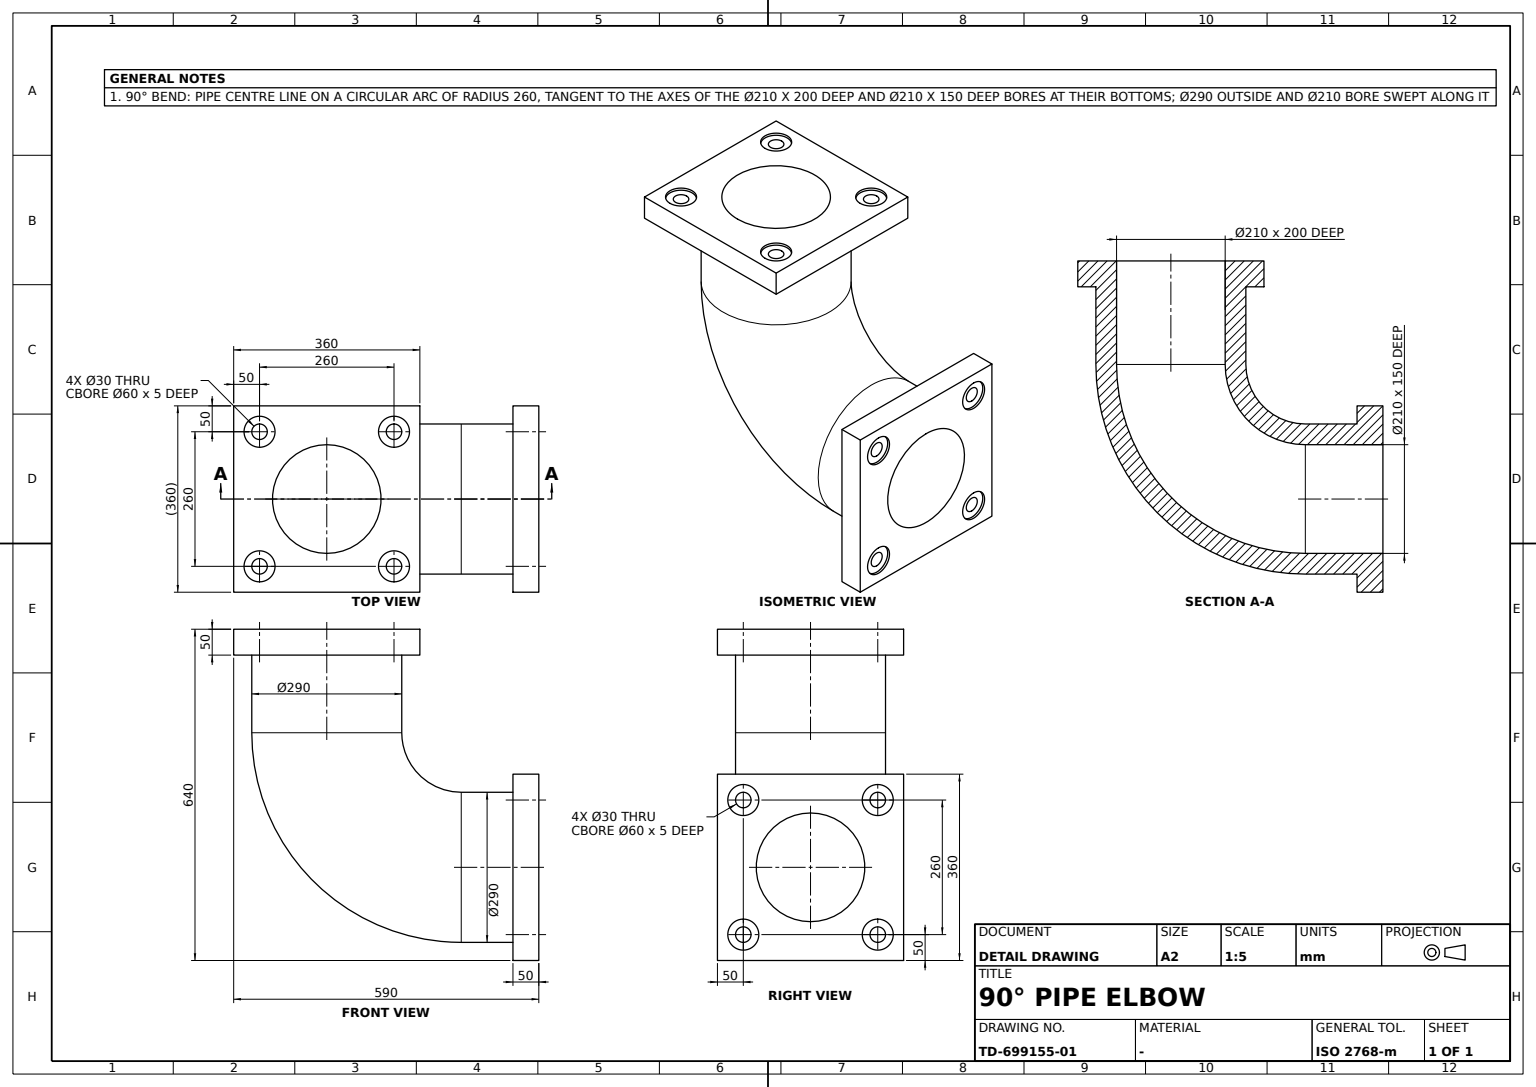
ISO-10303-21;
HEADER;
FILE_DESCRIPTION((''),'2;1');
FILE_NAME('','',(''),(''),'','','');
FILE_SCHEMA(('AUTOMOTIVE_DESIGN'));
ENDSEC;
DATA;
#1=APPLICATION_CONTEXT('');
#2=PRODUCT_CONTEXT('',#1,'mechanical');
#3=PRODUCT('','','',(#2));
#4=PRODUCT_DEFINITION_FORMATION('','',#3);
#5=PRODUCT_DEFINITION_CONTEXT('',#1,'design');
#6=PRODUCT_DEFINITION('','',#4,#5);
#7=PRODUCT_DEFINITION_SHAPE('','',#6);
#8=(LENGTH_UNIT()NAMED_UNIT(*)SI_UNIT(.MILLI.,.METRE.));
#9=(NAMED_UNIT(*)PLANE_ANGLE_UNIT()SI_UNIT($,.RADIAN.));
#10=(NAMED_UNIT(*)SI_UNIT($,.STERADIAN.)SOLID_ANGLE_UNIT());
#11=UNCERTAINTY_MEASURE_WITH_UNIT(LENGTH_MEASURE(0.005),#8,'distance_accuracy_value','');
#12=(GEOMETRIC_REPRESENTATION_CONTEXT(3)GLOBAL_UNCERTAINTY_ASSIGNED_CONTEXT((#11))GLOBAL_UNIT_ASSIGNED_CONTEXT((#8,#9,#10))REPRESENTATION_CONTEXT('',''));
#13=CARTESIAN_POINT('',(160.,-130.,460.));
#14=VERTEX_POINT('',#13);
#15=CARTESIAN_POINT('',(130.,-130.,460.));
#16=DIRECTION('',(0.,0.,1.));
#17=DIRECTION('',(1.,0.,0.));
#18=AXIS2_PLACEMENT_3D('',#15,#16,#17);
#19=CIRCLE('',#18,30.);
#20=EDGE_CURVE('',#14,#14,#19,.T.);
#21=ORIENTED_EDGE('',*,*,#20,.F.);
#22=EDGE_LOOP('',(#21));
#23=FACE_BOUND('',#22,.T.);
#24=CARTESIAN_POINT('',(105.,0.,460.));
#25=VERTEX_POINT('',#24);
#26=CARTESIAN_POINT('',(0.,0.,460.));
#27=AXIS2_PLACEMENT_3D('',#26,#16,#17);
#28=CIRCLE('',#27,105.);
#29=EDGE_CURVE('',#25,#25,#28,.T.);
#30=ORIENTED_EDGE('',*,*,#29,.F.);
#31=EDGE_LOOP('',(#30));
#32=FACE_BOUND('',#31,.T.);
#33=CARTESIAN_POINT('',(160.,130.,460.));
#34=VERTEX_POINT('',#33);
#35=CARTESIAN_POINT('',(130.,130.,460.));
#36=AXIS2_PLACEMENT_3D('',#35,#16,#17);
#37=CIRCLE('',#36,30.);
#38=EDGE_CURVE('',#34,#34,#37,.T.);
#39=ORIENTED_EDGE('',*,*,#38,.F.);
#40=EDGE_LOOP('',(#39));
#41=FACE_BOUND('',#40,.T.);
#42=CARTESIAN_POINT('',(-100.,130.,460.));
#43=VERTEX_POINT('',#42);
#44=CARTESIAN_POINT('',(-130.,130.,460.));
#45=AXIS2_PLACEMENT_3D('',#44,#16,#17);
#46=CIRCLE('',#45,30.);
#47=EDGE_CURVE('',#43,#43,#46,.T.);
#48=ORIENTED_EDGE('',*,*,#47,.F.);
#49=EDGE_LOOP('',(#48));
#50=FACE_BOUND('',#49,.T.);
#51=CARTESIAN_POINT('',(-180.,180.,460.));
#52=VERTEX_POINT('',#51);
#53=CARTESIAN_POINT('',(180.,180.,460.));
#54=VERTEX_POINT('',#53);
#55=CARTESIAN_POINT('',(0.,180.,460.));
#56=VECTOR('',#17,1000.);
#57=LINE('',#55,#56);
#58=EDGE_CURVE('',#52,#54,#57,.T.);
#59=ORIENTED_EDGE('',*,*,#58,.F.);
#60=CARTESIAN_POINT('',(-180.,-180.,460.));
#61=VERTEX_POINT('',#60);
#62=CARTESIAN_POINT('',(-180.,410.,460.));
#63=DIRECTION('',(0.,1.,0.));
#64=VECTOR('',#63,1000.);
#65=LINE('',#62,#64);
#66=EDGE_CURVE('',#61,#52,#65,.T.);
#67=ORIENTED_EDGE('',*,*,#66,.F.);
#68=CARTESIAN_POINT('',(180.,-180.,460.));
#69=VERTEX_POINT('',#68);
#70=CARTESIAN_POINT('',(0.,-180.,460.));
#71=DIRECTION('',(-1.,0.,0.));
#72=VECTOR('',#71,1000.);
#73=LINE('',#70,#72);
#74=EDGE_CURVE('',#69,#61,#73,.T.);
#75=ORIENTED_EDGE('',*,*,#74,.F.);
#76=CARTESIAN_POINT('',(180.,410.,460.));
#77=DIRECTION('',(0.,-1.,0.));
#78=VECTOR('',#77,1000.);
#79=LINE('',#76,#78);
#80=EDGE_CURVE('',#54,#69,#79,.T.);
#81=ORIENTED_EDGE('',*,*,#80,.F.);
#82=EDGE_LOOP('',(#59,#67,#75,#81));
#83=FACE_BOUND('',#82,.T.);
#84=CARTESIAN_POINT('',(-100.,-130.,460.));
#85=VERTEX_POINT('',#84);
#86=CARTESIAN_POINT('',(-130.,-130.,460.));
#87=AXIS2_PLACEMENT_3D('',#86,#16,#17);
#88=CIRCLE('',#87,30.);
#89=EDGE_CURVE('',#85,#85,#88,.T.);
#90=ORIENTED_EDGE('',*,*,#89,.F.);
#91=EDGE_LOOP('',(#90));
#92=FACE_BOUND('',#91,.T.);
#93=PLANE('',#27);
#94=ADVANCED_FACE('',(#23,#32,#41,#50,#83,#92),#93,.T.);
#95=CARTESIAN_POINT('',(-180.,410.,-180.));
#96=VERTEX_POINT('',#95);
#97=CARTESIAN_POINT('',(180.,410.,-180.));
#98=VERTEX_POINT('',#97);
#99=LINE('',#95,#56);
#100=EDGE_CURVE('',#96,#98,#99,.T.);
#101=ORIENTED_EDGE('',*,*,#100,.T.);
#102=CARTESIAN_POINT('',(180.,360.,-180.));
#103=VERTEX_POINT('',#102);
#104=LINE('',#97,#78);
#105=EDGE_CURVE('',#98,#103,#104,.T.);
#106=ORIENTED_EDGE('',*,*,#105,.T.);
#107=CARTESIAN_POINT('',(-180.,360.,-180.));
#108=VERTEX_POINT('',#107);
#109=LINE('',#107,#56);
#110=EDGE_CURVE('',#108,#103,#109,.T.);
#111=ORIENTED_EDGE('',*,*,#110,.F.);
#112=LINE('',#95,#78);
#113=EDGE_CURVE('',#96,#108,#112,.T.);
#114=ORIENTED_EDGE('',*,*,#113,.F.);
#115=EDGE_LOOP('',(#101,#106,#111,#114));
#116=FACE_BOUND('',#115,.T.);
#117=DIRECTION('',(0.,0.,-1.));
#118=AXIS2_PLACEMENT_3D('',#95,#117,#17);
#119=PLANE('',#118);
#120=ADVANCED_FACE('',(#116),#119,.T.);
#121=ORIENTED_EDGE('',*,*,#38,.T.);
#122=EDGE_LOOP('',(#121));
#123=FACE_BOUND('',#122,.T.);
#124=CARTESIAN_POINT('',(100.,130.,455.));
#125=VERTEX_POINT('',#124);
#126=CARTESIAN_POINT('',(130.,130.,455.));
#127=AXIS2_PLACEMENT_3D('',#126,#117,#71);
#128=CIRCLE('',#127,30.);
#129=EDGE_CURVE('',#125,#125,#128,.T.);
#130=ORIENTED_EDGE('',*,*,#129,.T.);
#131=EDGE_LOOP('',(#130));
#132=FACE_BOUND('',#131,.T.);
#133=CARTESIAN_POINT('',(130.,130.,459.9));
#134=AXIS2_PLACEMENT_3D('',#133,#117,#17);
#135=CYLINDRICAL_SURFACE('',#134,30.);
#136=ADVANCED_FACE('',(#123,#132),#135,.F.);
#137=CARTESIAN_POINT('',(115.,130.,410.));
#138=VERTEX_POINT('',#137);
#139=CARTESIAN_POINT('',(130.,130.,410.));
#140=AXIS2_PLACEMENT_3D('',#139,#117,#71);
#141=CIRCLE('',#140,15.);
#142=EDGE_CURVE('',#138,#138,#141,.T.);
#143=ORIENTED_EDGE('',*,*,#142,.T.);
#144=EDGE_LOOP('',(#143));
#145=FACE_BOUND('',#144,.T.);
#146=CARTESIAN_POINT('',(115.,130.,455.));
#147=VERTEX_POINT('',#146);
#148=CIRCLE('',#127,15.);
#149=EDGE_CURVE('',#147,#147,#148,.T.);
#150=ORIENTED_EDGE('',*,*,#149,.F.);
#151=EDGE_LOOP('',(#150));
#152=FACE_BOUND('',#151,.T.);
#153=CYLINDRICAL_SURFACE('',#134,15.);
#154=ADVANCED_FACE('',(#145,#152),#153,.F.);
#155=CARTESIAN_POINT('',(-130.,405.,-160.));
#156=VERTEX_POINT('',#155);
#157=CARTESIAN_POINT('',(-130.,405.,-130.));
#158=AXIS2_PLACEMENT_3D('',#157,#77,#117);
#159=CIRCLE('',#158,30.);
#160=EDGE_CURVE('',#156,#156,#159,.T.);
#161=ORIENTED_EDGE('',*,*,#160,.T.);
#162=EDGE_LOOP('',(#161));
#163=FACE_BOUND('',#162,.T.);
#164=CARTESIAN_POINT('',(-130.,410.,-100.));
#165=VERTEX_POINT('',#164);
#166=CARTESIAN_POINT('',(-130.,410.,-130.));
#167=AXIS2_PLACEMENT_3D('',#166,#63,#16);
#168=CIRCLE('',#167,30.);
#169=EDGE_CURVE('',#165,#165,#168,.T.);
#170=ORIENTED_EDGE('',*,*,#169,.T.);
#171=EDGE_LOOP('',(#170));
#172=FACE_BOUND('',#171,.T.);
#173=CARTESIAN_POINT('',(-130.,409.9,-130.));
#174=AXIS2_PLACEMENT_3D('',#173,#77,#17);
#175=CYLINDRICAL_SURFACE('',#174,30.);
#176=ADVANCED_FACE('',(#163,#172),#175,.F.);
#177=CARTESIAN_POINT('',(180.,410.,180.));
#178=VERTEX_POINT('',#177);
#179=VECTOR('',#16,1000.);
#180=LINE('',#97,#179);
#181=EDGE_CURVE('',#98,#178,#180,.T.);
#182=ORIENTED_EDGE('',*,*,#181,.T.);
#183=CARTESIAN_POINT('',(180.,360.,180.));
#184=VERTEX_POINT('',#183);
#185=LINE('',#177,#78);
#186=EDGE_CURVE('',#178,#184,#185,.T.);
#187=ORIENTED_EDGE('',*,*,#186,.T.);
#188=LINE('',#102,#179);
#189=EDGE_CURVE('',#103,#184,#188,.T.);
#190=ORIENTED_EDGE('',*,*,#189,.F.);
#191=ORIENTED_EDGE('',*,*,#105,.F.);
#192=EDGE_LOOP('',(#182,#187,#190,#191));
#193=FACE_BOUND('',#192,.T.);
#194=AXIS2_PLACEMENT_3D('',#97,#17,#16);
#195=PLANE('',#194);
#196=ADVANCED_FACE('',(#193),#195,.T.);
#197=CARTESIAN_POINT('',(0.,260.,105.));
#198=VERTEX_POINT('',#197);
#199=CARTESIAN_POINT('',(0.,260.,0.));
#200=AXIS2_PLACEMENT_3D('',#199,#63,#16);
#201=CIRCLE('',#200,105.);
#202=EDGE_CURVE('',#198,#198,#201,.T.);
#203=ORIENTED_EDGE('',*,*,#202,.F.);
#204=EDGE_LOOP('',(#203));
#205=FACE_BOUND('',#204,.T.);
#206=CARTESIAN_POINT('',(0.,410.,105.));
#207=VERTEX_POINT('',#206);
#208=CARTESIAN_POINT('',(0.,410.,0.));
#209=AXIS2_PLACEMENT_3D('',#208,#63,#16);
#210=CIRCLE('',#209,105.);
#211=EDGE_CURVE('',#207,#207,#210,.T.);
#212=ORIENTED_EDGE('',*,*,#211,.T.);
#213=EDGE_LOOP('',(#212));
#214=FACE_BOUND('',#213,.T.);
#215=CARTESIAN_POINT('',(0.,335.,0.));
#216=AXIS2_PLACEMENT_3D('',#215,#63,#71);
#217=CYLINDRICAL_SURFACE('',#216,105.);
#218=ADVANCED_FACE('',(#205,#214),#217,.F.);
#219=CARTESIAN_POINT('',(-160.,130.,455.));
#220=VERTEX_POINT('',#219);
#221=CARTESIAN_POINT('',(-130.,130.,455.));
#222=AXIS2_PLACEMENT_3D('',#221,#117,#71);
#223=CIRCLE('',#222,30.);
#224=EDGE_CURVE('',#220,#220,#223,.T.);
#225=ORIENTED_EDGE('',*,*,#224,.F.);
#226=EDGE_LOOP('',(#225));
#227=FACE_BOUND('',#226,.T.);
#228=CARTESIAN_POINT('',(-145.,130.,455.));
#229=VERTEX_POINT('',#228);
#230=CIRCLE('',#222,15.);
#231=EDGE_CURVE('',#229,#229,#230,.T.);
#232=ORIENTED_EDGE('',*,*,#231,.T.);
#233=EDGE_LOOP('',(#232));
#234=FACE_BOUND('',#233,.T.);
#235=CARTESIAN_POINT('',(145.,130.,455.));
#236=AXIS2_PLACEMENT_3D('',#235,#117,#17);
#237=PLANE('',#236);
#238=ADVANCED_FACE('',(#227,#234),#237,.F.);
#239=CARTESIAN_POINT('',(-160.,-130.,455.));
#240=VERTEX_POINT('',#239);
#241=CARTESIAN_POINT('',(-130.,-130.,455.));
#242=AXIS2_PLACEMENT_3D('',#241,#117,#71);
#243=CIRCLE('',#242,30.);
#244=EDGE_CURVE('',#240,#240,#243,.T.);
#245=ORIENTED_EDGE('',*,*,#244,.F.);
#246=EDGE_LOOP('',(#245));
#247=FACE_BOUND('',#246,.T.);
#248=CARTESIAN_POINT('',(-145.,-130.,455.));
#249=VERTEX_POINT('',#248);
#250=CIRCLE('',#242,15.);
#251=EDGE_CURVE('',#249,#249,#250,.T.);
#252=ORIENTED_EDGE('',*,*,#251,.T.);
#253=EDGE_LOOP('',(#252));
#254=FACE_BOUND('',#253,.T.);
#255=ADVANCED_FACE('',(#247,#254),#237,.F.);
#256=CARTESIAN_POINT('',(-180.,180.,410.));
#257=VERTEX_POINT('',#256);
#258=CARTESIAN_POINT('',(-180.,180.,180.));
#259=LINE('',#258,#179);
#260=EDGE_CURVE('',#257,#52,#259,.T.);
#261=ORIENTED_EDGE('',*,*,#260,.F.);
#262=CARTESIAN_POINT('',(-180.,-180.,410.));
#263=VERTEX_POINT('',#262);
#264=CARTESIAN_POINT('',(-180.,0.,410.));
#265=LINE('',#264,#64);
#266=EDGE_CURVE('',#263,#257,#265,.T.);
#267=ORIENTED_EDGE('',*,*,#266,.F.);
#268=LINE('',#262,#179);
#269=EDGE_CURVE('',#263,#61,#268,.T.);
#270=ORIENTED_EDGE('',*,*,#269,.T.);
#271=ORIENTED_EDGE('',*,*,#66,.T.);
#272=EDGE_LOOP('',(#261,#267,#270,#271));
#273=FACE_BOUND('',#272,.T.);
#274=CARTESIAN_POINT('',(-180.,410.,180.));
#275=AXIS2_PLACEMENT_3D('',#274,#71,#117);
#276=PLANE('',#275);
#277=ADVANCED_FACE('',(#273),#276,.T.);
#278=CARTESIAN_POINT('',(0.,260.,145.));
#279=VERTEX_POINT('',#278);
#280=CIRCLE('',#200,145.);
#281=EDGE_CURVE('',#279,#279,#280,.T.);
#282=ORIENTED_EDGE('',*,*,#281,.T.);
#283=EDGE_LOOP('',(#282));
#284=FACE_BOUND('',#283,.T.);
#285=CARTESIAN_POINT('',(0.,360.,145.));
#286=VERTEX_POINT('',#285);
#287=CARTESIAN_POINT('',(0.,360.,0.));
#288=AXIS2_PLACEMENT_3D('',#287,#63,#16);
#289=CIRCLE('',#288,145.);
#290=EDGE_CURVE('',#286,#286,#289,.T.);
#291=ORIENTED_EDGE('',*,*,#290,.F.);
#292=EDGE_LOOP('',(#291));
#293=FACE_BOUND('',#292,.T.);
#294=CYLINDRICAL_SURFACE('',#216,145.);
#295=ADVANCED_FACE('',(#284,#293),#294,.T.);
#296=CARTESIAN_POINT('',(-130.,405.,100.));
#297=VERTEX_POINT('',#296);
#298=CARTESIAN_POINT('',(-130.,405.,130.));
#299=AXIS2_PLACEMENT_3D('',#298,#77,#117);
#300=CIRCLE('',#299,30.);
#301=EDGE_CURVE('',#297,#297,#300,.T.);
#302=ORIENTED_EDGE('',*,*,#301,.T.);
#303=EDGE_LOOP('',(#302));
#304=FACE_BOUND('',#303,.T.);
#305=CARTESIAN_POINT('',(-130.,410.,160.));
#306=VERTEX_POINT('',#305);
#307=CARTESIAN_POINT('',(-130.,410.,130.));
#308=AXIS2_PLACEMENT_3D('',#307,#63,#16);
#309=CIRCLE('',#308,30.);
#310=EDGE_CURVE('',#306,#306,#309,.T.);
#311=ORIENTED_EDGE('',*,*,#310,.T.);
#312=EDGE_LOOP('',(#311));
#313=FACE_BOUND('',#312,.T.);
#314=CARTESIAN_POINT('',(-130.,409.9,130.));
#315=AXIS2_PLACEMENT_3D('',#314,#77,#17);
#316=CYLINDRICAL_SURFACE('',#315,30.);
#317=ADVANCED_FACE('',(#304,#313),#316,.F.);
#318=CARTESIAN_POINT('',(115.,-130.,455.));
#319=VERTEX_POINT('',#318);
#320=CARTESIAN_POINT('',(130.,-130.,455.));
#321=AXIS2_PLACEMENT_3D('',#320,#117,#71);
#322=CIRCLE('',#321,15.);
#323=EDGE_CURVE('',#319,#319,#322,.T.);
#324=ORIENTED_EDGE('',*,*,#323,.F.);
#325=EDGE_LOOP('',(#324));
#326=FACE_BOUND('',#325,.T.);
#327=CARTESIAN_POINT('',(115.,-130.,410.));
#328=VERTEX_POINT('',#327);
#329=CARTESIAN_POINT('',(130.,-130.,410.));
#330=AXIS2_PLACEMENT_3D('',#329,#117,#71);
#331=CIRCLE('',#330,15.);
#332=EDGE_CURVE('',#328,#328,#331,.T.);
#333=ORIENTED_EDGE('',*,*,#332,.T.);
#334=EDGE_LOOP('',(#333));
#335=FACE_BOUND('',#334,.T.);
#336=CARTESIAN_POINT('',(130.,-130.,459.9));
#337=AXIS2_PLACEMENT_3D('',#336,#117,#17);
#338=CYLINDRICAL_SURFACE('',#337,15.);
#339=ADVANCED_FACE('',(#326,#335),#338,.F.);
#340=CARTESIAN_POINT('',(130.,405.,-160.));
#341=VERTEX_POINT('',#340);
#342=CARTESIAN_POINT('',(130.,405.,-130.));
#343=AXIS2_PLACEMENT_3D('',#342,#77,#117);
#344=CIRCLE('',#343,30.);
#345=EDGE_CURVE('',#341,#341,#344,.T.);
#346=ORIENTED_EDGE('',*,*,#345,.T.);
#347=EDGE_LOOP('',(#346));
#348=FACE_BOUND('',#347,.T.);
#349=CARTESIAN_POINT('',(130.,410.,-100.));
#350=VERTEX_POINT('',#349);
#351=CARTESIAN_POINT('',(130.,410.,-130.));
#352=AXIS2_PLACEMENT_3D('',#351,#63,#16);
#353=CIRCLE('',#352,30.);
#354=EDGE_CURVE('',#350,#350,#353,.T.);
#355=ORIENTED_EDGE('',*,*,#354,.T.);
#356=EDGE_LOOP('',(#355));
#357=FACE_BOUND('',#356,.T.);
#358=CARTESIAN_POINT('',(130.,409.9,-130.));
#359=AXIS2_PLACEMENT_3D('',#358,#77,#17);
#360=CYLINDRICAL_SURFACE('',#359,30.);
#361=ADVANCED_FACE('',(#348,#357),#360,.F.);
#362=CARTESIAN_POINT('',(-130.,405.,-145.));
#363=VERTEX_POINT('',#362);
#364=CIRCLE('',#158,15.);
#365=EDGE_CURVE('',#363,#363,#364,.T.);
#366=ORIENTED_EDGE('',*,*,#365,.F.);
#367=EDGE_LOOP('',(#366));
#368=FACE_BOUND('',#367,.T.);
#369=CARTESIAN_POINT('',(-130.,360.,-115.));
#370=VERTEX_POINT('',#369);
#371=CARTESIAN_POINT('',(-130.,360.,-130.));
#372=AXIS2_PLACEMENT_3D('',#371,#63,#16);
#373=CIRCLE('',#372,15.);
#374=EDGE_CURVE('',#370,#370,#373,.T.);
#375=ORIENTED_EDGE('',*,*,#374,.F.);
#376=EDGE_LOOP('',(#375));
#377=FACE_BOUND('',#376,.T.);
#378=CYLINDRICAL_SURFACE('',#174,15.);
#379=ADVANCED_FACE('',(#368,#377),#378,.F.);
#380=ORIENTED_EDGE('',*,*,#323,.T.);
#381=EDGE_LOOP('',(#380));
#382=FACE_BOUND('',#381,.T.);
#383=CARTESIAN_POINT('',(100.,-130.,455.));
#384=VERTEX_POINT('',#383);
#385=CIRCLE('',#321,30.);
#386=EDGE_CURVE('',#384,#384,#385,.T.);
#387=ORIENTED_EDGE('',*,*,#386,.F.);
#388=EDGE_LOOP('',(#387));
#389=FACE_BOUND('',#388,.T.);
#390=ADVANCED_FACE('',(#382,#389),#237,.F.);
#391=CARTESIAN_POINT('',(130.,360.,145.));
#392=VERTEX_POINT('',#391);
#393=CARTESIAN_POINT('',(130.,360.,130.));
#394=AXIS2_PLACEMENT_3D('',#393,#63,#16);
#395=CIRCLE('',#394,15.);
#396=EDGE_CURVE('',#392,#392,#395,.T.);
#397=ORIENTED_EDGE('',*,*,#396,.F.);
#398=EDGE_LOOP('',(#397));
#399=FACE_BOUND('',#398,.T.);
#400=CARTESIAN_POINT('',(130.,405.,115.));
#401=VERTEX_POINT('',#400);
#402=CARTESIAN_POINT('',(130.,405.,130.));
#403=AXIS2_PLACEMENT_3D('',#402,#77,#117);
#404=CIRCLE('',#403,15.);
#405=EDGE_CURVE('',#401,#401,#404,.T.);
#406=ORIENTED_EDGE('',*,*,#405,.F.);
#407=EDGE_LOOP('',(#406));
#408=FACE_BOUND('',#407,.T.);
#409=CARTESIAN_POINT('',(130.,409.9,130.));
#410=AXIS2_PLACEMENT_3D('',#409,#77,#17);
#411=CYLINDRICAL_SURFACE('',#410,15.);
#412=ADVANCED_FACE('',(#399,#408),#411,.F.);
#413=ORIENTED_EDGE('',*,*,#244,.T.);
#414=EDGE_LOOP('',(#413));
#415=FACE_BOUND('',#414,.T.);
#416=ORIENTED_EDGE('',*,*,#89,.T.);
#417=EDGE_LOOP('',(#416));
#418=FACE_BOUND('',#417,.T.);
#419=CARTESIAN_POINT('',(-130.,-130.,459.9));
#420=AXIS2_PLACEMENT_3D('',#419,#117,#17);
#421=CYLINDRICAL_SURFACE('',#420,30.);
#422=ADVANCED_FACE('',(#415,#418),#421,.F.);
#423=ORIENTED_EDGE('',*,*,#224,.T.);
#424=EDGE_LOOP('',(#423));
#425=FACE_BOUND('',#424,.T.);
#426=ORIENTED_EDGE('',*,*,#47,.T.);
#427=EDGE_LOOP('',(#426));
#428=FACE_BOUND('',#427,.T.);
#429=CARTESIAN_POINT('',(-130.,130.,459.9));
#430=AXIS2_PLACEMENT_3D('',#429,#117,#17);
#431=CYLINDRICAL_SURFACE('',#430,30.);
#432=ADVANCED_FACE('',(#425,#428),#431,.F.);
#433=CARTESIAN_POINT('',(-145.,130.,410.));
#434=VERTEX_POINT('',#433);
#435=CARTESIAN_POINT('',(-130.,130.,410.));
#436=AXIS2_PLACEMENT_3D('',#435,#117,#71);
#437=CIRCLE('',#436,15.);
#438=EDGE_CURVE('',#434,#434,#437,.T.);
#439=ORIENTED_EDGE('',*,*,#438,.T.);
#440=EDGE_LOOP('',(#439));
#441=FACE_BOUND('',#440,.T.);
#442=ORIENTED_EDGE('',*,*,#231,.F.);
#443=EDGE_LOOP('',(#442));
#444=FACE_BOUND('',#443,.T.);
#445=CYLINDRICAL_SURFACE('',#430,15.);
#446=ADVANCED_FACE('',(#441,#444),#445,.F.);
#447=CARTESIAN_POINT('',(180.,180.,410.));
#448=VERTEX_POINT('',#447);
#449=CARTESIAN_POINT('',(180.,-180.,410.));
#450=VERTEX_POINT('',#449);
#451=CARTESIAN_POINT('',(180.,0.,410.));
#452=LINE('',#451,#78);
#453=EDGE_CURVE('',#448,#450,#452,.T.);
#454=ORIENTED_EDGE('',*,*,#453,.F.);
#455=LINE('',#447,#179);
#456=EDGE_CURVE('',#448,#54,#455,.T.);
#457=ORIENTED_EDGE('',*,*,#456,.T.);
#458=ORIENTED_EDGE('',*,*,#80,.T.);
#459=CARTESIAN_POINT('',(180.,-180.,-180.));
#460=LINE('',#459,#179);
#461=EDGE_CURVE('',#450,#69,#460,.T.);
#462=ORIENTED_EDGE('',*,*,#461,.F.);
#463=EDGE_LOOP('',(#454,#457,#458,#462));
#464=FACE_BOUND('',#463,.T.);
#465=ADVANCED_FACE('',(#464),#195,.T.);
#466=CARTESIAN_POINT('',(-130.,360.,145.));
#467=VERTEX_POINT('',#466);
#468=CARTESIAN_POINT('',(-130.,360.,130.));
#469=AXIS2_PLACEMENT_3D('',#468,#63,#16);
#470=CIRCLE('',#469,15.);
#471=EDGE_CURVE('',#467,#467,#470,.T.);
#472=ORIENTED_EDGE('',*,*,#471,.T.);
#473=EDGE_LOOP('',(#472));
#474=FACE_BOUND('',#473,.T.);
#475=ORIENTED_EDGE('',*,*,#374,.T.);
#476=EDGE_LOOP('',(#475));
#477=FACE_BOUND('',#476,.T.);
#478=CARTESIAN_POINT('',(-180.,360.,180.));
#479=VERTEX_POINT('',#478);
#480=LINE('',#183,#72);
#481=EDGE_CURVE('',#184,#479,#480,.T.);
#482=ORIENTED_EDGE('',*,*,#481,.T.);
#483=VECTOR('',#117,1000.);
#484=LINE('',#478,#483);
#485=EDGE_CURVE('',#479,#108,#484,.T.);
#486=ORIENTED_EDGE('',*,*,#485,.T.);
#487=ORIENTED_EDGE('',*,*,#110,.T.);
#488=ORIENTED_EDGE('',*,*,#189,.T.);
#489=EDGE_LOOP('',(#482,#486,#487,#488));
#490=FACE_BOUND('',#489,.T.);
#491=ORIENTED_EDGE('',*,*,#396,.T.);
#492=EDGE_LOOP('',(#491));
#493=FACE_BOUND('',#492,.T.);
#494=ORIENTED_EDGE('',*,*,#290,.T.);
#495=EDGE_LOOP('',(#494));
#496=FACE_BOUND('',#495,.T.);
#497=CARTESIAN_POINT('',(130.,360.,-115.));
#498=VERTEX_POINT('',#497);
#499=CARTESIAN_POINT('',(130.,360.,-130.));
#500=AXIS2_PLACEMENT_3D('',#499,#63,#16);
#501=CIRCLE('',#500,15.);
#502=EDGE_CURVE('',#498,#498,#501,.T.);
#503=ORIENTED_EDGE('',*,*,#502,.T.);
#504=EDGE_LOOP('',(#503));
#505=FACE_BOUND('',#504,.T.);
#506=AXIS2_PLACEMENT_3D('',#287,#63,#71);
#507=PLANE('',#506);
#508=ADVANCED_FACE('',(#474,#477,#490,#493,#496,#505),#507,.F.);
#509=ORIENTED_EDGE('',*,*,#251,.F.);
#510=EDGE_LOOP('',(#509));
#511=FACE_BOUND('',#510,.T.);
#512=CARTESIAN_POINT('',(-145.,-130.,410.));
#513=VERTEX_POINT('',#512);
#514=CARTESIAN_POINT('',(-130.,-130.,410.));
#515=AXIS2_PLACEMENT_3D('',#514,#117,#71);
#516=CIRCLE('',#515,15.);
#517=EDGE_CURVE('',#513,#513,#516,.T.);
#518=ORIENTED_EDGE('',*,*,#517,.T.);
#519=EDGE_LOOP('',(#518));
#520=FACE_BOUND('',#519,.T.);
#521=CYLINDRICAL_SURFACE('',#420,15.);
#522=ADVANCED_FACE('',(#511,#520),#521,.F.);
#523=ORIENTED_EDGE('',*,*,#160,.F.);
#524=EDGE_LOOP('',(#523));
#525=FACE_BOUND('',#524,.T.);
#526=ORIENTED_EDGE('',*,*,#365,.T.);
#527=EDGE_LOOP('',(#526));
#528=FACE_BOUND('',#527,.T.);
#529=CARTESIAN_POINT('',(-115.,405.,130.));
#530=AXIS2_PLACEMENT_3D('',#529,#77,#17);
#531=PLANE('',#530);
#532=ADVANCED_FACE('',(#525,#528),#531,.F.);
#533=CARTESIAN_POINT('',(-145.,0.,260.));
#534=VERTEX_POINT('',#533);
#535=CARTESIAN_POINT('',(0.,0.,260.));
#536=AXIS2_PLACEMENT_3D('',#535,#117,#71);
#537=CIRCLE('',#536,145.);
#538=EDGE_CURVE('',#534,#534,#537,.T.);
#539=ORIENTED_EDGE('',*,*,#538,.F.);
#540=EDGE_LOOP('',(#539));
#541=FACE_BOUND('',#540,.T.);
#542=CARTESIAN_POINT('',(-145.,0.,410.));
#543=VERTEX_POINT('',#542);
#544=CARTESIAN_POINT('',(0.,0.,410.));
#545=AXIS2_PLACEMENT_3D('',#544,#117,#71);
#546=CIRCLE('',#545,145.);
#547=EDGE_CURVE('',#543,#543,#546,.T.);
#548=ORIENTED_EDGE('',*,*,#547,.T.);
#549=EDGE_LOOP('',(#548));
#550=FACE_BOUND('',#549,.T.);
#551=CARTESIAN_POINT('',(0.,0.,335.));
#552=AXIS2_PLACEMENT_3D('',#551,#117,#71);
#553=CYLINDRICAL_SURFACE('',#552,145.);
#554=ADVANCED_FACE('',(#541,#550),#553,.T.);
#555=CARTESIAN_POINT('',(130.,405.,-145.));
#556=VERTEX_POINT('',#555);
#557=CIRCLE('',#343,15.);
#558=EDGE_CURVE('',#556,#556,#557,.T.);
#559=ORIENTED_EDGE('',*,*,#558,.F.);
#560=EDGE_LOOP('',(#559));
#561=FACE_BOUND('',#560,.T.);
#562=ORIENTED_EDGE('',*,*,#502,.F.);
#563=EDGE_LOOP('',(#562));
#564=FACE_BOUND('',#563,.T.);
#565=CYLINDRICAL_SURFACE('',#359,15.);
#566=ADVANCED_FACE('',(#561,#564),#565,.F.);
#567=ORIENTED_EDGE('',*,*,#471,.F.);
#568=EDGE_LOOP('',(#567));
#569=FACE_BOUND('',#568,.T.);
#570=CARTESIAN_POINT('',(-130.,405.,115.));
#571=VERTEX_POINT('',#570);
#572=CIRCLE('',#299,15.);
#573=EDGE_CURVE('',#571,#571,#572,.T.);
#574=ORIENTED_EDGE('',*,*,#573,.F.);
#575=EDGE_LOOP('',(#574));
#576=FACE_BOUND('',#575,.T.);
#577=CYLINDRICAL_SURFACE('',#315,15.);
#578=ADVANCED_FACE('',(#569,#576),#577,.F.);
#579=VERTEX_POINT('',#274);
#580=LINE('',#274,#78);
#581=EDGE_CURVE('',#579,#479,#580,.T.);
#582=ORIENTED_EDGE('',*,*,#581,.F.);
#583=LINE('',#274,#483);
#584=EDGE_CURVE('',#579,#96,#583,.T.);
#585=ORIENTED_EDGE('',*,*,#584,.T.);
#586=ORIENTED_EDGE('',*,*,#113,.T.);
#587=ORIENTED_EDGE('',*,*,#485,.F.);
#588=EDGE_LOOP('',(#582,#585,#586,#587));
#589=FACE_BOUND('',#588,.T.);
#590=ADVANCED_FACE('',(#589),#276,.T.);
#591=ORIENTED_EDGE('',*,*,#20,.T.);
#592=EDGE_LOOP('',(#591));
#593=FACE_BOUND('',#592,.T.);
#594=ORIENTED_EDGE('',*,*,#386,.T.);
#595=EDGE_LOOP('',(#594));
#596=FACE_BOUND('',#595,.T.);
#597=CYLINDRICAL_SURFACE('',#337,30.);
#598=ADVANCED_FACE('',(#593,#596),#597,.F.);
#599=ORIENTED_EDGE('',*,*,#438,.F.);
#600=EDGE_LOOP('',(#599));
#601=FACE_BOUND('',#600,.T.);
#602=LINE('',#449,#72);
#603=EDGE_CURVE('',#450,#263,#602,.T.);
#604=ORIENTED_EDGE('',*,*,#603,.T.);
#605=ORIENTED_EDGE('',*,*,#266,.T.);
#606=LINE('',#256,#56);
#607=EDGE_CURVE('',#257,#448,#606,.T.);
#608=ORIENTED_EDGE('',*,*,#607,.T.);
#609=ORIENTED_EDGE('',*,*,#453,.T.);
#610=EDGE_LOOP('',(#604,#605,#608,#609));
#611=FACE_BOUND('',#610,.T.);
#612=ORIENTED_EDGE('',*,*,#547,.F.);
#613=EDGE_LOOP('',(#612));
#614=FACE_BOUND('',#613,.T.);
#615=ORIENTED_EDGE('',*,*,#142,.F.);
#616=EDGE_LOOP('',(#615));
#617=FACE_BOUND('',#616,.T.);
#618=ORIENTED_EDGE('',*,*,#332,.F.);
#619=EDGE_LOOP('',(#618));
#620=FACE_BOUND('',#619,.T.);
#621=ORIENTED_EDGE('',*,*,#517,.F.);
#622=EDGE_LOOP('',(#621));
#623=FACE_BOUND('',#622,.T.);
#624=PLANE('',#545);
#625=ADVANCED_FACE('',(#601,#611,#614,#617,#620,#623),#624,.T.);
#626=ORIENTED_EDGE('',*,*,#603,.F.);
#627=ORIENTED_EDGE('',*,*,#461,.T.);
#628=ORIENTED_EDGE('',*,*,#74,.T.);
#629=ORIENTED_EDGE('',*,*,#269,.F.);
#630=EDGE_LOOP('',(#626,#627,#628,#629));
#631=FACE_BOUND('',#630,.T.);
#632=AXIS2_PLACEMENT_3D('',#449,#63,#71);
#633=PLANE('',#632);
#634=ADVANCED_FACE('',(#631),#633,.F.);
#635=ORIENTED_EDGE('',*,*,#186,.F.);
#636=LINE('',#177,#72);
#637=EDGE_CURVE('',#178,#579,#636,.T.);
#638=ORIENTED_EDGE('',*,*,#637,.T.);
#639=ORIENTED_EDGE('',*,*,#581,.T.);
#640=ORIENTED_EDGE('',*,*,#481,.F.);
#641=EDGE_LOOP('',(#635,#638,#639,#640));
#642=FACE_BOUND('',#641,.T.);
#643=AXIS2_PLACEMENT_3D('',#177,#16,#71);
#644=PLANE('',#643);
#645=ADVANCED_FACE('',(#642),#644,.T.);
#646=ORIENTED_EDGE('',*,*,#169,.F.);
#647=EDGE_LOOP('',(#646));
#648=FACE_BOUND('',#647,.T.);
#649=ORIENTED_EDGE('',*,*,#211,.F.);
#650=EDGE_LOOP('',(#649));
#651=FACE_BOUND('',#650,.T.);
#652=ORIENTED_EDGE('',*,*,#637,.F.);
#653=ORIENTED_EDGE('',*,*,#181,.F.);
#654=ORIENTED_EDGE('',*,*,#100,.F.);
#655=ORIENTED_EDGE('',*,*,#584,.F.);
#656=EDGE_LOOP('',(#652,#653,#654,#655));
#657=FACE_BOUND('',#656,.T.);
#658=ORIENTED_EDGE('',*,*,#354,.F.);
#659=EDGE_LOOP('',(#658));
#660=FACE_BOUND('',#659,.T.);
#661=ORIENTED_EDGE('',*,*,#310,.F.);
#662=EDGE_LOOP('',(#661));
#663=FACE_BOUND('',#662,.T.);
#664=CARTESIAN_POINT('',(130.,410.,160.));
#665=VERTEX_POINT('',#664);
#666=CARTESIAN_POINT('',(130.,410.,130.));
#667=AXIS2_PLACEMENT_3D('',#666,#63,#16);
#668=CIRCLE('',#667,30.);
#669=EDGE_CURVE('',#665,#665,#668,.T.);
#670=ORIENTED_EDGE('',*,*,#669,.F.);
#671=EDGE_LOOP('',(#670));
#672=FACE_BOUND('',#671,.T.);
#673=AXIS2_PLACEMENT_3D('',#208,#63,#71);
#674=PLANE('',#673);
#675=ADVANCED_FACE('',(#648,#651,#657,#660,#663,#672),#674,.T.);
#676=ORIENTED_EDGE('',*,*,#607,.F.);
#677=ORIENTED_EDGE('',*,*,#260,.T.);
#678=ORIENTED_EDGE('',*,*,#58,.T.);
#679=ORIENTED_EDGE('',*,*,#456,.F.);
#680=EDGE_LOOP('',(#676,#677,#678,#679));
#681=FACE_BOUND('',#680,.T.);
#682=AXIS2_PLACEMENT_3D('',#256,#77,#17);
#683=PLANE('',#682);
#684=ADVANCED_FACE('',(#681),#683,.F.);
#685=ORIENTED_EDGE('',*,*,#129,.F.);
#686=EDGE_LOOP('',(#685));
#687=FACE_BOUND('',#686,.T.);
#688=ORIENTED_EDGE('',*,*,#149,.T.);
#689=EDGE_LOOP('',(#688));
#690=FACE_BOUND('',#689,.T.);
#691=ADVANCED_FACE('',(#687,#690),#237,.F.);
#692=ORIENTED_EDGE('',*,*,#29,.T.);
#693=EDGE_LOOP('',(#692));
#694=FACE_BOUND('',#693,.T.);
#695=CARTESIAN_POINT('',(105.,0.,260.));
#696=VERTEX_POINT('',#695);
#697=AXIS2_PLACEMENT_3D('',#535,#16,#17);
#698=CIRCLE('',#697,105.);
#699=EDGE_CURVE('',#696,#696,#698,.F.);
#700=ORIENTED_EDGE('',*,*,#699,.T.);
#701=EDGE_LOOP('',(#700));
#702=FACE_BOUND('',#701,.T.);
#703=CARTESIAN_POINT('',(0.,0.,435.));
#704=AXIS2_PLACEMENT_3D('',#703,#16,#17);
#705=CYLINDRICAL_SURFACE('',#704,105.);
#706=ADVANCED_FACE('',(#694,#702),#705,.F.);
#707=ORIENTED_EDGE('',*,*,#301,.F.);
#708=EDGE_LOOP('',(#707));
#709=FACE_BOUND('',#708,.T.);
#710=ORIENTED_EDGE('',*,*,#573,.T.);
#711=EDGE_LOOP('',(#710));
#712=FACE_BOUND('',#711,.T.);
#713=ADVANCED_FACE('',(#709,#712),#531,.F.);
#714=ORIENTED_EDGE('',*,*,#699,.F.);
#715=EDGE_LOOP('',(#714));
#716=FACE_BOUND('',#715,.T.);
#717=ORIENTED_EDGE('',*,*,#202,.T.);
#718=EDGE_LOOP('',(#717));
#719=FACE_BOUND('',#718,.T.);
#720=CARTESIAN_POINT('',(0.,260.,260.));
#721=AXIS2_PLACEMENT_3D('',#720,#17,#77);
#722=TOROIDAL_SURFACE('',#721,260.,105.);
#723=ADVANCED_FACE('',(#716,#719),#722,.F.);
#724=ORIENTED_EDGE('',*,*,#345,.F.);
#725=EDGE_LOOP('',(#724));
#726=FACE_BOUND('',#725,.T.);
#727=ORIENTED_EDGE('',*,*,#558,.T.);
#728=EDGE_LOOP('',(#727));
#729=FACE_BOUND('',#728,.T.);
#730=ADVANCED_FACE('',(#726,#729),#531,.F.);
#731=CARTESIAN_POINT('',(130.,405.,100.));
#732=VERTEX_POINT('',#731);
#733=CIRCLE('',#403,30.);
#734=EDGE_CURVE('',#732,#732,#733,.T.);
#735=ORIENTED_EDGE('',*,*,#734,.T.);
#736=EDGE_LOOP('',(#735));
#737=FACE_BOUND('',#736,.T.);
#738=ORIENTED_EDGE('',*,*,#669,.T.);
#739=EDGE_LOOP('',(#738));
#740=FACE_BOUND('',#739,.T.);
#741=CYLINDRICAL_SURFACE('',#410,30.);
#742=ADVANCED_FACE('',(#737,#740),#741,.F.);
#743=ORIENTED_EDGE('',*,*,#538,.T.);
#744=EDGE_LOOP('',(#743));
#745=FACE_BOUND('',#744,.T.);
#746=ORIENTED_EDGE('',*,*,#281,.F.);
#747=EDGE_LOOP('',(#746));
#748=FACE_BOUND('',#747,.T.);
#749=TOROIDAL_SURFACE('',#721,260.,145.);
#750=ADVANCED_FACE('',(#745,#748),#749,.T.);
#751=ORIENTED_EDGE('',*,*,#405,.T.);
#752=EDGE_LOOP('',(#751));
#753=FACE_BOUND('',#752,.T.);
#754=ORIENTED_EDGE('',*,*,#734,.F.);
#755=EDGE_LOOP('',(#754));
#756=FACE_BOUND('',#755,.T.);
#757=ADVANCED_FACE('',(#753,#756),#531,.F.);
#758=CLOSED_SHELL('',(#94,#120,#136,#154,#176,#196,#218,#238,#255,#277,#295,#317,#339,#361,#379,#390,#412,#422,#432,#446,#465,#508,#522,#532,#554,#566,#578,#590,#598,#625,#634,#645,#675,#684,#691,#706,#713,#723,#730,#742,#750,#757));
#759=MANIFOLD_SOLID_BREP('',#758);
#760=ADVANCED_BREP_SHAPE_REPRESENTATION('',(#759),#12);
#761=SHAPE_DEFINITION_REPRESENTATION(#7,#760);
ENDSEC;
END-ISO-10303-21;
